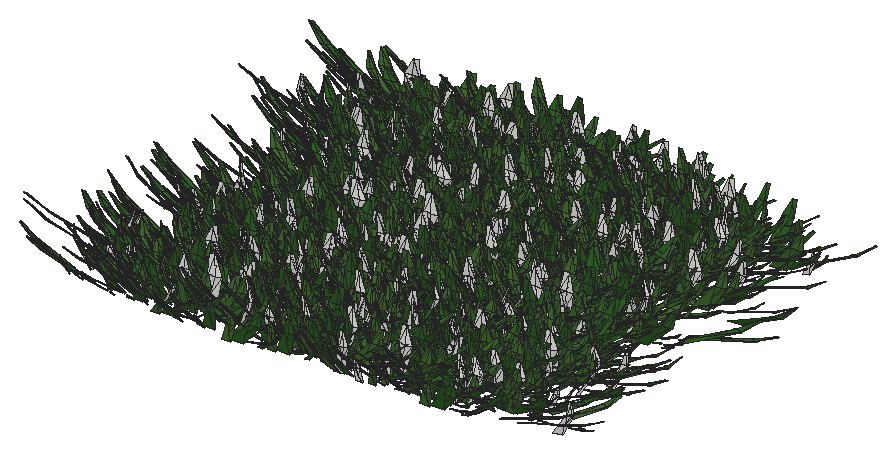
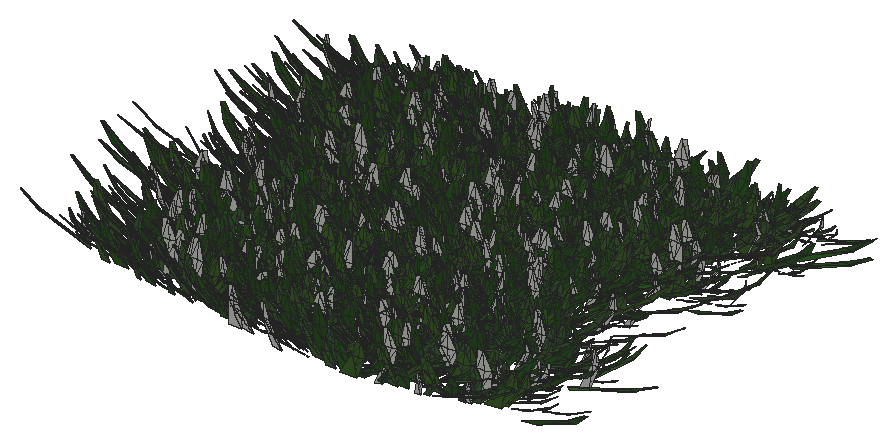
# SketchUp Ruby script. Lengths in inches.
U = 1.inch
M = Sketchup.active_model
def pt(a) = Geom::Point3d.new(a.map { |v| v * U })
def face(e, loops, mat)
  f = e.add_face(loops[0].map { |a| pt(a) })
  loops[1..].each { |l| e.add_face(l.map { |a| pt(a) }).erase! }
  f.material = f.back_material = mat if mat
  f
end
# faces: each face lists its corners as indices into pts; further lists are holes
def faces(e, pts, list, mat = nil) = list.each { |f| face(e, (f[0].is_a?(Array) ? f : [f]).map { |l| l.map { |i| pts[i] } }, mat) }
# xy, xz, yz: faces in a plane at the given z, y or x. An outline is a flat list of corners, or four numbers for a rectangle; further outlines are holes
def ring(l) = l.size == 4 ? [[l[0], l[1]], [l[2], l[1]], [l[2], l[3]], [l[0], l[3]]] : l.each_slice(2).to_a
def flat(e, list, mat, &to3) = list.each { |f| face(e, (f[0].is_a?(Array) ? f : [f]).map { |l| ring(l).map { |u, v| to3.(u, v) } }, mat) }
def xy(e, z, list, mat = nil) = flat(e, list, mat) { |x, y| [x, y, z] }
def xz(e, y, list, mat = nil) = flat(e, list, mat) { |x, z| [x, y, z] }
def yz(e, x, list, mat = nil) = flat(e, list, mat) { |y, z| [x, y, z] }
def lines(e, pts, list) = list.each { |a, b| e.add_line(pt(pts[a]), pt(pts[b])) }
# prism: a flat outline (further loops are holes) pulled along v
def prism(e, loops, v, mat = nil)
  f = face(e, loops, mat); d = Geom::Vector3d.new(v.map { |x| x * U })
  f.pushpull(f.normal.samedirection?(d) ? d.length : -d.length)
end
def box(e, o, s, mat = nil) = prism(e, [[o, [o[0] + s[0], o[1], o[2]], [o[0] + s[0], o[1] + s[1], o[2]], [o[0], o[1] + s[1], o[2]]]], [0, 0, s[2]], mat)
def at(x, y, z, deg = 0) = Geom::Transformation.translation(pt([x, y, z])) * Geom::Transformation.rotation(ORIGIN, Z_AXIS, deg.degrees)
def axes(o, x, y, z) = Geom::Transformation.new([*x, 0, *y, 0, *z, 0, *pt(o).to_a, 1])
def part(name) = M.definitions.add(name)
# library, detail: a bought-in or finely detailed component or shape, given as its bounding box
def library(name, o, s) = part(name).tap { |d| box(d.entities, o, s) }
def detail(e, o, s) = box(e.add_group.entities, o, s)
def put(e, d, t, mat = nil) = e.add_instance(d, t).tap { |i| i.material = mat if mat }
def group(e, t, mat = nil) = e.add_group.tap { |g| g.transformation = t; g.material = mat if mat }.entities
root = M.entities
M.materials.add("Material10").color = [48, 100, 38]
M.materials.add("Material3").color = [68, 110, 58]
M.materials.add("Material4").color = [48, 90, 38]
M.materials.add("Material5").color = [68, 110, 48]
M.materials.add("Material6").color = [48, 90, 48]
M.materials.add("Material7").color = [58, 110, 58]
M.materials.add("Material8").color = [58, 90, 38]
M.materials.add("Material9").color = [68, 100, 58]
c1 = part("grass00")
p = [[-0.6875,0.15,0],[-0.56,0.08,5.52],[-0.04,0.03,2.76],[0.48,-0.02,0],[0.35,-0.02,5.52],[-0.1,-0.14,5.52],
  [-0.12,0.65,8.37],[-0.42,0.65,8.37]]
faces(c1.entities,p,[[0,1,2,3],[3,2,4],[1,5,2],[5,4,2],[1,6,5],[4,5,6],[7,6,1]])
c2 = part("Group16\#1")
put(c2.entities,c1,axes([1.44,-0.61,-0.01],[0.05352,0.12609,0],[-0.10704,0.04543,0.07239],[0.06664,-0.02828,0.11628]),"Material6")
put(c2.entities,c1,axes([0.76,-0.15,-0.01],[0.04676,0.24062,0],[-0.23162,0.04501,0.06642],[0.0652,-0.01267,0.23595]),"Material3")
put(c2.entities,c1,axes([0.79,0.01,-0.01],[-0.00606,0.34651,0],[-0.34381,-0.00602,0.0432],[0.04319,0.00076,0.34386]))
put(c2.entities,c1,axes([1,0.23,-0.01],[-0.07192,0.31144,0],[-0.28722,-0.06632,0.1236],[0.12043,0.02781,0.29478]),"Material5")
put(c2.entities,c1,axes([1.66,0.77,-0.01],[-0.13828,0.29651,0],[-0.21551,-0.1005,0.22471],[0.20365,0.09498,0.23779]),"Material10")
put(c2.entities,c1,axes([0.6875,0.52,-0.01],[-0.18126,0.24051,0],[-0.22746,-0.17142,0.09788],[0.07817,0.05891,0.28481]),"Material5")
put(c2.entities,c1,axes([0.68,0.78,-0.01],[-0.215,0.18688,0],[-0.12385,-0.14248,0.21334],[0.13995,0.16101,0.18878]),"Material3")
put(c2.entities,c1,axes([0.56,1,-0.01],[-0.13756,0.07624,0],[-0.06159,-0.11112,0.0927],[0.04494,0.08108,0.12705]),"Material5")
put(c2.entities,c1,axes([0.2,0.64,-0.01],[-0.23729,0.07254,0],[-0.05711,-0.18681,0.153],[0.04473,0.14632,0.19535]),"Material10")
put(c2.entities,c1,axes([0.0625,0.72,-0.01],[-0.28874,0.02525,0],[-0.02179,-0.24916,0.14647],[0.01276,0.14591,0.25012]),"Material3")
put(c2.entities,c1,axes([-0.08,0.62,-0.01],[-0.34089,-0.04187,0],[0.03255,-0.26504,0.216],[-0.02633,0.21439,0.26703]),"Material10")
put(c2.entities,c1,axes([-0.34,0.98,-0.01],[-0.14314,-0.0493,0],[0.04397,-0.12769,0.06843],[-0.02228,0.0647,0.13505]),"Material10")
put(c2.entities,c1,axes([-0.87,1.45,-0.01],[-0.23488,-0.14114,0],[0.13761,-0.22901,0.06087],[-0.03135,0.05217,0.26717]))
put(c2.entities,c1,axes([-0.72,0.77,-0.01],[-0.14208,-0.13251,0],[0.07209,-0.0773,0.16301],[-0.11118,0.11922,0.1057]),"Material10")
put(c2.entities,c1,axes([-0.62,0.43,-0.01],[-0.14845,-0.21203,0],[0.18654,-0.13061,0.12304],[-0.10079,0.07057,0.22772]),"Material3")
put(c2.entities,c1,axes([-0.68,0.29,-0.01],[-0.13639,-0.32136,0],[0.31723,-0.13464,0.05579],[-0.05136,0.0218,0.34462]),"Material4")
put(c2.entities,c1,axes([-0.64,0.125,-0.01],[-0.0458,-0.23569,0],[0.22124,-0.043,0.08276],[-0.08124,0.01579,0.22538]),"Material7")
put(c2.entities,c1,axes([-1.6,-0.03,-0.01],[0.00576,-0.32897,0],[0.27526,0.00482,0.18018],[-0.18015,-0.00315,0.2753]),"Material5")
put(c2.entities,c1,axes([-1.36,-0.31,-0.01],[0.05718,-0.24765,0],[0.18172,0.04196,0.17267],[-0.16825,-0.03885,0.1865]),"Material10")
put(c2.entities,c1,axes([-1.54,-0.72,-0.01],[0.06537,-0.14017,0],[0.13555,0.06321,0.03939],[-0.0357,-0.01665,0.14956]))
put(c2.entities,c1,axes([-1.19,-0.9,-0.01],[0.09597,-0.12735,0],[0.11214,0.08451,0.07557],[-0.06035,-0.04548,0.14042]),"Material9")
put(c2.entities,c1,axes([-0.47,-0.54,-0.01],[0.11588,-0.10072,0],[0.0618,0.0711,0.12124],[-0.07953,-0.0915,0.0942]))
put(c2.entities,c1,axes([-0.47,-0.84,-0.01],[0.11927,-0.0661,0],[0.06603,0.11913,0.00646],[-0.00313,-0.00565,0.13621]),"Material5")
put(c2.entities,c1,axes([-0.38,-1.24,-0.01],[0.28037,-0.08571,0],[0.0618,0.20215,0.20315],[-0.05939,-0.19428,0.21139]),"Material9")
put(c2.entities,c1,axes([-0.06,-0.66,-0.01],[0.22719,-0.01987,0],[0.01247,0.14255,0.17758],[-0.01547,-0.17691,0.1431]),"Material8")
put(c2.entities,c1,axes([0.11,-0.89,-0.01],[0.14882,0.01828,0],[-0.01058,0.08611,0.12229],[0.01491,-0.12138,0.08676]),"Material6")
put(c2.entities,c1,axes([0.25,-0.72,-0.01],[0.20481,0.07053,0],[-0.06206,0.18022,0.10291],[0.03351,-0.0973,0.1906]),"Material6")
put(c2.entities,c1,axes([0.85,-1.42,-0.01],[0.16481,0.09904,0],[-0.09472,0.15762,0.05616],[0.02893,-0.04814,0.18389]),"Material5")
put(c2.entities,c1,axes([1.01,-1.09,-0.01],[0.21858,0.20385,0],[-0.17495,0.1876,0.15339],[0.10462,-0.11218,0.25652]),"Material10")
put(c2.entities,c1,axes([1.01,-0.71,-0.01],[0.08733,0.12473,0],[-0.06445,0.04512,0.13037],[0.1068,-0.07477,0.07867]),"Material6")
c3 = part("Group15\#1")
put(c3.entities,c2,at(0,0,0))
c4 = part("3darcstudiotree_grass00\#1")
put(c4.entities,c3,at(0,0,0))
put(root,c4,axes([26.93,16.5,7.6],[-1.46443,-0.98467,0],[4.53365,-0.42141,-0.02925],[0.15457,-0.01437,1.7044]))
put(root,c4,axes([26.97,8.6,7.6],[-4.82729,-0.45997,0],[1.31646,-0.86349,-0.04688],[0.11487,-0.07535,1.58936]))
put(root,c4,axes([27.1,9.74,7.6],[-5.02983,-0.31612,0],[0.92163,-0.91652,-0.02201],[0.03056,-0.03039,1.34565]))
put(root,c4,axes([27.39,33.84,7.6],[-1.60248,-1.17219,0],[4.18284,-0.35739,-0.03013],[0.15857,-0.01355,1.53631]))
put(root,c4,axes([26,3.94,7.6],[4,0,0],[0,1,0],[0,0,1]))
put(root,c4,axes([26.25,33.12,7.6],[3.56901,0.48429,0],[-2.2351,1.02948,-0.01651],[-0.0487,0.02243,1.81134]))
put(root,c4,axes([27.1,17.92,7.6],[-2.03185,0.95693,0],[-3.64296,-0.48344,-0.02935],[-0.13306,-0.01766,1.32321]))
put(root,c4,axes([26.98,40.27,7.6],[-2.36821,1.01615,0],[-4.30311,-0.62679,-0.00219],[-0.01,-0.00146,1.64693]))
put(root,c4,axes([27.15,11.93,7.6],[3.55456,-0.14349,0],[0.62802,0.97236,-0.03713],[0.03348,0.05184,1.39317]))
put(root,c4,axes([27.5625,31.14,7.6],[3.6372,-0.13455,0],[0.71258,1.2039,-0.00326],[0.00297,0.00501,1.88794]))
put(root,c4,axes([27.4375,5.4,7.6],[1.65013,1.13441,0],[-3.55007,0.32275,-0.03897],[-0.23777,0.02162,1.53286]))
put(root,c4,axes([29.72,35.81,7.6],[-5.16631,0.09452,0],[-0.34124,-1.1657,-0.0067],[-0.00219,-0.00748,1.30916]))
put(root,c4,axes([29.61,40.29,7.6],[0.40076,-1.15293,0],[4.50783,0.09793,-0.03115],[0.17233,0.00374,1.5702]))
put(root,c4,axes([30.21,37.21,7.6],[1.18754,-1.01824,0],[3.81557,0.27812,-0.01207],[0.07759,0.00566,1.66287]))
put(root,c4,axes([30.46,5.8,7.6],[2.49255,-0.69469,0],[3.67207,0.82346,-0.03873],[0.17763,0.03983,1.89965]))
put(root,c4,axes([30.98,26.54,7.6],[-3.93651,0.31096,0],[-1.27927,-1.01217,-0.02199],[-0.03758,-0.02973,1.50537]))
put(root,c4,axes([30.96,23.63,7.6],[2.99864,-0.87357,0],[3.91675,0.8403,-0.00643],[0.02559,0.00549,1.6911]))
put(root,c4,axes([30.2,38.51,7.6],[-0.4238,1.09775,0],[-5.15842,-0.12447,-0.01578],[-0.06645,-0.0016,1.37044]))
put(root,c4,axes([30.26,16.4,7.6],[0.74164,0.96677,0],[-4.8523,0.23265,-0.00068],[-0.00352,0.00017,1.62852]))
put(root,c4,axes([31.85,29.28,7.6],[1.73951,-1.15891,0],[3.52233,0.33044,-0.02337],[0.15547,0.01459,1.67088]))
put(root,c4,axes([32.25,8.09,7.6],[-4.02575,0.06277,0],[-0.3115,-1.24857,-0.0193],[-0.00513,-0.02057,1.33558]))
put(root,c4,axes([31.11,7.24,7.6],[0.21868,1.00492,0],[-3.69218,0.05022,-0.03311],[-0.20682,0.00281,1.44579]))
put(root,c4,axes([32.62,41.94,7.6],[0.06879,-0.93707,0],[3.83645,0.0176,-0.01436],[0.09429,0.00043,1.57494]))
put(root,c4,axes([31.73,9.48,7.6],[-2.74984,0.77403,0],[-3.3377,-0.7411,-0.01682],[-0.07048,-0.01565,1.56312]))
put(root,c4,axes([32.74,33.01,7.6],[-3.8395,0.24007,0],[-0.9565,-0.9561,-0.00789],[-0.01338,-0.01337,1.7222]))
put(root,c4,axes([31.52,11.96,7.6],[4.9283,0.10353,0],[-0.353,1.05028,-0.00911],[-0.00564,0.01678,1.94776]))
put(root,c4,axes([32.87,28.41,7.6],[-3.40628,0.74927,0],[-2.81528,-0.79992,-0.02195],[-0.09915,-0.02817,1.82186]))
put(root,c4,axes([33.375,31.71,7.6],[2.93374,-0.98597,0],[4.11982,0.76616,-0.01386],[0.04525,0.00841,1.30579]))
put(root,c4,axes([34,20.78,7.6],[-4.41204,-0.22693,0],[0.9521,-1.15695,-0.02294],[0.02698,-0.03278,1.72347]))
put(root,c4,axes([32.92,17.62,7.6],[3.69247,-0.55992,0],[2.62164,1.08055,-0.03972],[0.1072,0.04419,1.6444]))
put(root,c4,axes([32.07,34.09,7.6],[3.49468,0.70982,0],[-2.50295,0.77018,-0.0068],[-0.02397,0.00738,1.38619]))
put(root,c4,axes([32.16,22.05,7.6],[0.58267,1.0863,0],[-4.76439,0.15972,-0.0098],[-0.05571,0.00187,1.72283]))
put(root,c4,axes([32.3,25.43,7.6],[4.02178,0.69197,0],[-2.67404,0.97136,-0.05897],[-0.21681,0.07876,1.91169]))
put(root,c4,axes([33.72,13.98,7.6],[-3.59564,0.7993,0],[-2.95427,-0.83061,-0.01814],[-0.07531,-0.02117,1.73642]))
put(root,c4,axes([33.86,19.39,7.6],[-3.02071,0.81725,0],[-3.67065,-0.84796,-0.01856],[-0.08057,-0.01861,1.84646]))
put(root,c4,axes([33.44,3.98,7.6],[4.41696,-0.08184,0],[0.31192,1.05211,-0.02045],[0.01033,0.03484,1.8024]))
put(root,c4,axes([33.96,13.41,7.6],[1.69404,0.9375,0],[-3.93647,0.44457,-0.01637],[-0.07596,0.00858,1.37485]))
put(root,c4,axes([35.68,37.11,7.6],[-1.11853,-1.11565,0],[3.68055,-0.23063,-0.0349],[0.26302,-0.01648,1.84282]))
put(root,c4,axes([36.8,10.01,7.6],[-4.81712,-0.05846,0],[0.24162,-1.24435,-0.01036],[0.00226,-0.01162,1.39846]))
put(root,c4,axes([37.17,28.54,7.6],[-2.48915,-0.80051,0],[3.17734,-0.61749,-0.04864],[0.28827,-0.05602,1.88819]))
put(root,c4,axes([37.15,15.86,7.6],[-0.29922,-0.96853,0],[4.43417,-0.08562,-0.04603],[0.2662,-0.00514,1.61216]))
put(root,c4,axes([36.59,42.28,7.6],[-3.61794,0.71954,0],[-3.11711,-0.97958,-0.00639],[-0.02051,-0.00644,1.6128]))
put(root,c4,axes([37.68,30.2,7.6],[-4.63349,-0.14284,0],[0.49364,-1.00082,-0.03319],[0.02506,-0.0508,1.55524]))
put(root,c4,axes([38.02,39.86,7.6],[-1.47695,-1.05774,0],[4.67611,-0.40809,-0.05387],[0.24046,-0.02099,1.46363]))
put(root,c4,axes([36.56,22.01,7.6],[3.90451,-0.09036,0],[0.41259,1.1143,-0.05657],[0.02788,0.07529,1.49576]))
put(root,c4,axes([37.45,23.38,7.6],[-3.34722,0.62533,0],[-2.16221,-0.72335,-0.01872],[-0.08063,-0.02697,1.62421]))
put(root,c4,axes([37.66,7.36,7.6],[-3.49291,0.22015,0],[-1.20974,-1.19959,-0.01943],[-0.02054,-0.02037,1.33771]))
put(root,c4,axes([38.27,32.39,7.6],[-3.43835,-0.52535,0],[2.21532,-0.90619,-0.04274],[0.13952,-0.05707,1.66217]))
put(root,c4,axes([38.4,35.58,7.6],[-4.50993,0.04391,0],[-0.14231,-0.91361,-0.00954],[-0.0023,-0.01475,1.41434]))
put(root,c4,axes([37.44,34.04,7.6],[-0.6796,1.05515,0],[-3.94798,-0.15893,-0.03829],[-0.25732,-0.01036,1.70109]))
put(root,c4,axes([38.98,26.6,7.6],[-0.97949,-1.15886,0],[4.63427,-0.24481,-0.02196],[0.13062,-0.0069,1.79942]))
put(root,c4,axes([37.03,20.16,7.6],[3.07159,0.54643,0],[-2.5154,0.88372,-0.00585],[-0.0211,0.00741,1.68777]))
put(root,c4,axes([38.59,11.97,7.6],[1.11882,-0.9865,0],[3.53965,0.2509,-0.01712],[0.10104,0.00716,1.41054]))
put(root,c4,axes([39.42,19.625,7.6],[-4.7616,-0.19084,0],[0.68375,-1.06626,-0.05495],[0.05173,-0.08067,1.60563]))
put(root,c4,axes([39.03,42.98,7.6],[1.85003,-0.9013,0],[4.03488,0.51763,-0.0206],[0.11343,0.01455,1.75423]))
put(root,c4,axes([39.27,25.14,7.6],[0.8852,-0.96568,0],[4.22844,0.24225,-0.01662],[0.10834,0.00621,1.81323]))
put(root,c4,axes([37.97,18,7.6],[1.94137,0.91072,0],[-3.56961,0.47558,-0.05193],[-0.33599,0.04476,1.85357]))
put(root,c4,axes([39.66,30.66,7.6],[0.57898,-1.02169,0],[3.84832,0.1363,-0.02485],[0.19995,0.00708,1.97391]))
put(root,c4,axes([39.54,5.12,7.6],[3.44867,-0.28659,0],[1.33447,1.00364,-0.00205],[0.00439,0.0033,1.79239]))
put(root,c4,axes([39.63,8.35,7.6],[-1.8497,1.19261,0],[-4.37152,-0.42376,-0.03012],[-0.17466,-0.01693,1.82227]))
put(root,c4,axes([39.48,38.52,7.6],[2.87995,0.68544,0],[-2.96423,0.77841,-0.04733],[-0.16011,0.04205,1.31836]))
put(root,c4,axes([39.87,12.5,7.6],[2.68329,1.05589,0],[-3.47416,0.55179,-0.05376],[-0.29931,0.04754,1.69687]))
put(root,c4,axes([39.95,14.58,7.6],[4.3739,0.41815,0],[-1.70618,1.11543,-0.01506],[-0.02757,0.01802,1.52965]))
put(root,c4,axes([41.97,9.875,7.6],[-3.49233,-0.69736,0],[2.36447,-0.74006,-0.04095],[0.19015,-0.05951,1.76156]))
put(root,c4,axes([42.06,11.14,7.6],[2.09244,-0.94675,0],[3.21681,0.44435,-0.00396],[0.02932,0.00405,1.94458]))
put(root,c4,axes([42.15,13.33,7.6],[-4.33677,0.62867,0],[-2.01573,-0.86908,-0.01457],[-0.03892,-0.01678,1.33777]))
put(root,c4,axes([42.38,32.95,7.6],[-1.57293,1.10474,0],[-4.19735,-0.37351,-0.05045],[-0.27865,-0.0248,1.63245]))
put(root,c4,axes([43.95,18.69,7.6],[-1.17133,-0.98272,0],[4.80109,-0.35766,-0.01047],[0.05653,-0.00421,1.7643]))
put(root,c4,axes([41.97,34.09,7.6],[1.98106,1.05685,0],[-3.80639,0.44594,-0.0367],[-0.25209,0.02953,1.99296]))
put(root,c4,axes([43.62,5.53,7.6],[-3.60106,-0.04271,0],[0.19063,-1.00459,-0.03298],[0.01167,-0.06151,1.87797]))
put(root,c4,axes([43.78,40.21,7.6],[-0.42773,-1.06924,0],[4.56175,-0.11405,-0.04439],[0.21496,-0.00537,1.39437]))
put(root,c4,axes([43.8,21.82,7.6],[-3.73728,-0.2351,0],[0.93348,-0.92746,-0.02412],[0.03985,-0.03959,1.61843]))
put(root,c4,axes([44.22,26.37,7.6],[-3.21626,-0.41381,0],[2.3246,-1.12922,-0.00712],[0.01691,-0.00821,1.64666]))
put(root,c4,axes([43.65,27.66,7.6],[-3.61281,0.55884,0],[-2.43371,-0.98335,-0.03047],[-0.07699,-0.03111,1.38852]))
put(root,c4,axes([42.94,39.18,7.6],[4.54148,-0.35569,0],[1.42907,1.14041,-0.0458],[0.08138,0.06494,1.7756]))
put(root,c4,axes([42.59,7.9,7.6],[3.58951,0.93345,0],[-2.76207,0.66383,-0.03508],[-0.16897,0.04061,1.59982]))
put(root,c4,axes([43.82,6.62,7.6],[2.4755,-0.8869,0],[3.51902,0.61389,-0.05108],[0.27994,0.04883,1.79238]))
put(root,c4,axes([43.39,31.08,7.6],[-1.7461,0.91224,0],[-4.28122,-0.51216,-0.03408],[-0.14069,-0.01683,1.35762]))
put(root,c4,axes([44.96,29.24,7.6],[-0.33514,-1.12345,0],[4.93469,-0.09201,-0.02024],[0.12034,-0.00224,1.84439]))
put(root,c4,axes([44.05,23.36,7.6],[3.73698,-0.82778,0],[3.1181,0.87978,-0.01442],[0.06211,0.01752,1.90876]))
put(root,c4,axes([43.6875,20.3,7.6],[-2.06798,0.88983,0],[-4.26064,-0.61886,-0.00809],[-0.04346,-0.00631,1.91363]))
put(root,c4,axes([44.34,41.7,7.6],[3.27706,-0.90756,0],[3.76471,0.84961,-0.0538],[0.17294,0.03903,1.37259]))
put(root,c4,axes([44.14,16.4375,7.6],[3.50587,-0.21147,0],[1.00871,1.0452,-0.01591],[0.01836,0.01902,1.32206]))
put(root,c4,axes([45.59,37.0625,7.6],[0.8013,-1.18093,0],[4.91736,0.20854,-0.00997],[0.04679,0.00198,1.48373]))
put(root,c4,axes([44.91,17.25,7.6],[-2.9418,0.84861,0],[-3.1669,-0.68615,-0.03703],[-0.16978,-0.03678,1.58908]))
put(root,c4,axes([44.07,35.45,7.6],[1.17878,0.99592,0],[-4.61929,0.34171,-0.04809],[-0.20938,0.01549,1.36712]))
put(root,c4,axes([44.21,14.23,7.6],[4.48137,0.06994,0],[-0.29564,1.18401,-0.00965],[-0.00318,0.01276,1.57035]))
put(root,c4,axes([45.79,25.39,7.6],[3.67211,-0.34396,0],[1.33384,0.89,-0.02122],[0.05893,0.03932,1.88089]))
put(root,c4,axes([47.95,34.14,7.6],[-3.47348,-0.25295,0],[1.42263,-1.22094,-0.03129],[0.05076,-0.04356,1.8441]))
put(root,c4,axes([48.14,24.83,7.6],[-3.84564,-0.10505,0],[0.54072,-1.23711,-0.01667],[0.01042,-0.02384,1.79039]))
put(root,c4,axes([48.63,17.66,7.6],[-4.66165,0.25618,0],[-0.8902,-1.01241,-0.01858],[-0.02067,-0.02351,1.34303]))
put(root,c4,axes([49.14,8.3125,7.6],[-2.97895,-0.70139,0],[3.1973,-0.84873,-0.03536],[0.14976,-0.03975,1.8008]))
put(root,c4,axes([48.01,21.14,7.6],[-1.07038,1.23184,0],[-4.14964,-0.22536,-0.03052],[-0.1562,-0.00848,1.38983]))
put(root,c4,axes([47.97,27.91,7.6],[-0.92876,0.98956,0],[-4.3525,-0.25532,-0.03302],[-0.17329,-0.01017,1.5061]))
put(root,c4,axes([49.45,7.47,7.6],[1.90431,-1.19182,0],[3.88687,0.38816,-0.05078],[0.31147,0.0311,1.72798]))
put(root,c4,axes([48.57,5.48,7.6],[1.39207,0.89707,0],[-3.84824,0.37323,-0.02781],[-0.15819,0.01534,1.57422]))
put(root,c4,axes([50.19,24.04,7.6],[1.63221,-0.89951,0],[4.40071,0.49908,-0.00454],[0.01782,0.00202,1.30224]))
put(root,c4,axes([48.85,12.84,7.6],[3.72343,0.03185,0],[-0.16951,1.23856,-0.02332],[-0.00466,0.03402,1.80921]))
put(root,c4,axes([48.59,37.71,7.6],[1.62948,0.92472,0],[-3.84092,0.42301,-0.02705],[-0.14541,0.01601,1.54111]))
put(root,c4,axes([50.46,39.78,7.6],[-3.80407,0.33391,0],[-1.34486,-0.95759,-0.01418],[-0.0336,-0.02392,1.8149]))
put(root,c4,axes([49.11,32.43,7.6],[1.17856,0.89964,0],[-4.07228,0.33342,-0.00037],[-0.00182,0.00015,1.37352]))
put(root,c4,axes([50.98,19.1875,7.6],[-5.01358,0.24268,0],[-0.96954,-1.25187,-0.01839],[-0.01653,-0.02135,1.50803]))
put(root,c4,axes([51.23,10.97,7.6],[-1.78221,-0.81561,0],[4.04221,-0.55204,-0.05959],[0.23708,-0.03238,1.30502]))
put(root,c4,axes([50.38,31.18,7.6],[1.94348,-0.80631,0],[3.13656,0.47251,-0.04784],[0.31182,0.04697,1.7418]))
put(root,c4,axes([51.38,35.46,7.6],[-0.42607,-0.90558,0],[3.98828,-0.11728,-0.01277],[0.06985,-0.00205,1.38207]))
put(root,c4,axes([49.79,29.93,7.6],[0.24379,1.1856,0],[-4.61569,0.05932,-0.0387],[-0.22912,0.00294,1.71236]))
put(root,c4,axes([49.6,21.93,7.6],[1.54067,1.02539,0],[-4.80438,0.45117,-0.05425],[-0.27305,0.02564,1.72469]))
put(root,c4,axes([50.07,42.05,7.6],[4.09786,-0.28438,0],[1.1228,1.01119,-0.05393],[0.0997,0.08979,1.81331]))
put(root,c4,axes([50.64,9.8,7.6],[-1.78772,1.13511,0],[-3.81437,-0.37546,-0.00571],[-0.03781,-0.00372,1.8245]))
put(root,c4,axes([50.86,16.36,7.6],[-1.04195,1.21147,0],[-4.05734,-0.2181,-0.03186],[-0.23525,-0.01265,1.95913]))
put(root,c4,axes([52.01,38.93,7.6],[3.57558,-0.28511,0],[1.52231,1.19319,-0.05774],[0.1071,0.08395,1.91123]))
put(root,c4,axes([51.83,27.12,7.6],[3.07334,0.62938,0],[-2.31014,0.70504,-0.00694],[-0.03076,0.00939,1.5947]))
put(root,c4,axes([52.07,14.99,7.6],[5.00659,0.06984,0],[-0.21528,0.96462,-0.03032],[-0.01077,0.04826,1.54015]))
put(root,c4,axes([53.92,38.86,7.6],[-3.4834,-0.28364,0],[1.48287,-1.13821,-0.00123],[0.00249,-0.00191,1.95221]))
put(root,c4,axes([54.83,14.51,7.6],[-2.38105,-0.91178,0],[4.30884,-0.70326,-0.04707],[0.17067,-0.02786,1.39282]))
put(root,c4,axes([54.43,8.4,7.6],[-3.6738,0.0712,0],[-0.31805,-1.02562,-0.03359],[-0.01978,-0.06378,1.95875]))
put(root,c4,axes([54.04,29.72,7.6],[3.57103,-0.64395,0],[2.64716,0.9175,-0.00659],[0.02668,0.00925,1.95827]))
put(root,c4,axes([53.8125,5.88,7.6],[4.29662,-0.26643,0],[1.12646,1.13536,-0.04456],[0.05263,0.05304,1.43455]))
put(root,c4,axes([55.64,26.42,7.6],[-3.55163,-0.42804,0],[1.6107,-0.8353,-0.00927],[0.03461,-0.01795,1.99366]))
put(root,c4,axes([56.24,12.79,7.6],[-1.0061,-0.89228,0],[4.92324,-0.34695,-0.01485],[0.08067,-0.00569,1.80381]))
put(root,c4,axes([55.46,22.04,7.6],[0.65893,-0.95794,0],[4.25403,0.18289,-0.05034],[0.326,0.01402,1.77282]))
put(root,c4,axes([54.76,6.98,7.6],[4.30831,-0.62309,0],[2.18452,0.94404,-0.042],[0.12053,0.05209,1.56273]))
put(root,c4,axes([54.95,41.4375,7.6],[-1.21684,0.90717,0],[-3.63046,-0.30436,-0.03292],[-0.25254,-0.02117,1.93659]))
put(root,c4,axes([56.42,30.98,7.6],[-1.67207,-0.91895,0],[3.50462,-0.39855,-0.03768],[0.25255,-0.02872,1.77164]))
put(root,c4,axes([55.43,34.73,7.6],[-1.13491,0.99621,0],[-4.4644,-0.31787,-0.05457],[-0.24954,-0.01777,1.37935]))
put(root,c4,axes([56.8,35.77,7.6],[-3.91405,-0.00229,0],[0.01024,-1.09429,-0.04252],[0.00062,-0.06673,1.71753]))
put(root,c4,axes([56.48,33.18,7.6],[1.60501,-1.19589,0],[4.41908,0.37068,-0.04434],[0.27906,0.02341,1.93394]))
put(root,c4,axes([55.2,20.01,7.6],[3.60857,0.48959,0],[-2.46007,1.13325,-0.00178],[-0.00354,0.00163,1.34491]))
put(root,c4,axes([57.28,11.07,7.6],[-4.32765,0.00867,0],[-0.03775,-1.17772,-0.00779],[-0.00036,-0.01131,1.71052]))
put(root,c4,axes([55.72,39.71,7.6],[0.93736,0.93245,0],[-4.81106,0.30227,-0.04255],[-0.20854,0.0131,1.5668]))
put(root,c4,axes([56.87,16.17,7.6],[2.90531,-0.67717,0],[3.51467,0.94245,-0.02398],[0.07004,0.01878,1.37951]))
put(root,c4,axes([55.96,27.69,7.6],[-0.09714,1.01662,0],[-4.47384,-0.02672,-0.0357],[-0.18312,-0.00109,1.43525]))
put(root,c4,axes([56.67,18.56,7.6],[-1.68892,1.07101,0],[-4.3391,-0.42766,-0.03242],[-0.20319,-0.02003,1.96368]))
put(root,c4,axes([57.61,9.91,7.6],[1.59366,-0.94661,0],[3.67989,0.3872,-0.00467],[0.02447,0.00258,1.41828]))
put(root,c4,axes([57.03,36.74,7.6],[3.286,-0.8357,0],[2.84385,0.69888,-0.02297],[0.11018,0.02708,1.67632]))
put(root,c4,axes([58.13,17.2,7.6],[-4.44666,-0.20996,0],[0.93231,-1.23409,-0.03943],[0.03763,-0.04981,1.61444]))
put(root,c4,axes([56.47,25.32,7.6],[5.15116,-0.12991,0],[0.48402,1.19956,-0.01121],[0.00488,0.0121,1.30781]))
put(root,c4,axes([57.42,23.91,7.6],[4.97159,0.14622,0],[-0.54256,1.15298,-0.02625],[-0.02079,0.04418,1.96735]))
put(root,c4,axes([59.8,8.28,7.6],[-3.82917,-0.57908,0],[2.69029,-1.11185,-0.00291],[0.00714,-0.00295,1.54121]))
put(root,c4,axes([59.98,14.43,7.6],[1.08411,-0.99343,0],[4.41709,0.30127,-0.01691],[0.09138,0.00623,1.6028]))
put(root,c4,axes([60.08,30.9,7.6],[2.20022,-0.75251,0],[4.00552,0.73197,-0.0361],[0.16943,0.03096,1.80295]))
put(root,c4,axes([59.91,40.33,7.6],[-2.48301,0.65721,0],[-3.57154,-0.84335,-0.01576],[-0.06998,-0.01652,1.87507]))
